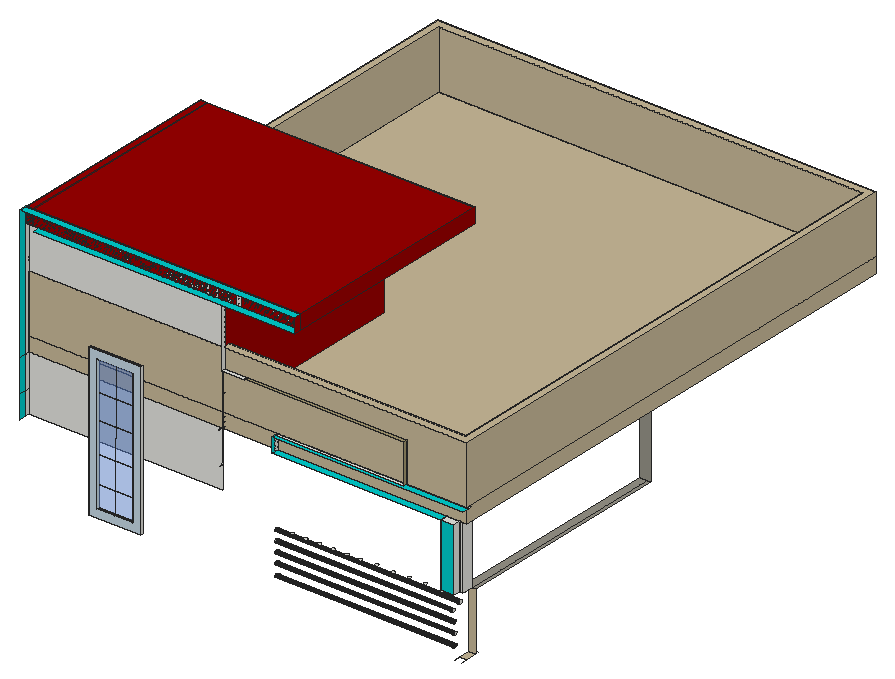
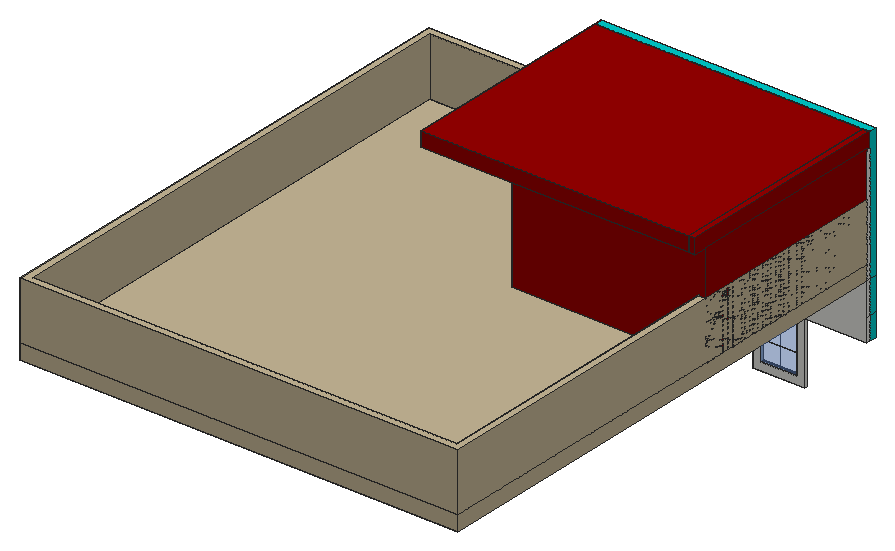
# SketchUp Ruby script. Lengths in inches.
U = 1.inch
M = Sketchup.active_model
def pt(a) = Geom::Point3d.new(a.map { |v| v * U })
def face(e, loops, mat)
  f = e.add_face(loops[0].map { |a| pt(a) })
  loops[1..].each { |l| e.add_face(l.map { |a| pt(a) }).erase! }
  f.material = f.back_material = mat if mat
  f
end
# faces: each face lists its corners as indices into pts; further lists are holes
def faces(e, pts, list, mat = nil) = list.each { |f| face(e, (f[0].is_a?(Array) ? f : [f]).map { |l| l.map { |i| pts[i] } }, mat) }
# xy, xz, yz: faces in a plane at the given z, y or x. An outline is a flat list of corners, or four numbers for a rectangle; further outlines are holes
def ring(l) = l.size == 4 ? [[l[0], l[1]], [l[2], l[1]], [l[2], l[3]], [l[0], l[3]]] : l.each_slice(2).to_a
def flat(e, list, mat, &to3) = list.each { |f| face(e, (f[0].is_a?(Array) ? f : [f]).map { |l| ring(l).map { |u, v| to3.(u, v) } }, mat) }
def xy(e, z, list, mat = nil) = flat(e, list, mat) { |x, y| [x, y, z] }
def xz(e, y, list, mat = nil) = flat(e, list, mat) { |x, z| [x, y, z] }
def yz(e, x, list, mat = nil) = flat(e, list, mat) { |y, z| [x, y, z] }
def lines(e, pts, list) = list.each { |a, b| e.add_line(pt(pts[a]), pt(pts[b])) }
# prism: a flat outline (further loops are holes) pulled along v
def prism(e, loops, v, mat = nil)
  f = face(e, loops, mat); d = Geom::Vector3d.new(v.map { |x| x * U })
  f.pushpull(f.normal.samedirection?(d) ? d.length : -d.length)
end
def box(e, o, s, mat = nil) = prism(e, [[o, [o[0] + s[0], o[1], o[2]], [o[0] + s[0], o[1] + s[1], o[2]], [o[0], o[1] + s[1], o[2]]]], [0, 0, s[2]], mat)
def at(x, y, z, deg = 0) = Geom::Transformation.translation(pt([x, y, z])) * Geom::Transformation.rotation(ORIGIN, Z_AXIS, deg.degrees)
def axes(o, x, y, z) = Geom::Transformation.new([*x, 0, *y, 0, *z, 0, *pt(o).to_a, 1])
def part(name) = M.definitions.add(name)
# library, detail: a bought-in or finely detailed component or shape, given as its bounding box
def library(name, o, s) = part(name).tap { |d| box(d.entities, o, s) }
def detail(e, o, s) = box(e.add_group.entities, o, s)
def put(e, d, t, mat = nil) = e.add_instance(d, t).tap { |i| i.material = mat if mat }
def group(e, t, mat = nil) = e.add_group.tap { |g| g.transformation = t; g.material = mat if mat }.entities
root = M.entities
M.materials.add("[Color A07]").color = [153, 0, 0]
M.materials.add("[Color B03]").color = [255, 140, 101]
M.materials.add("[Color H06]").color = [0, 204, 204]
M.materials.add("[Formica Beige]").color = [211, 187, 149]
M.materials.add("[Formica Graystone]").color = [149, 146, 135]
M.materials.add("[Quartz Light Brown]").color = [199, 184, 152]
M.materials.add("[Terrazzo Light Blue]").color = [196, 214, 227]
M.materials.add("[Translucent Glass Blue]").color = [100, 149, 237]
M.materials["[Translucent Glass Blue]"].alpha = 0.5
M.materials.add("[Translucent Glass Gray]1").color = [128, 128, 128]
M.materials["[Translucent Glass Gray]1"].alpha = 0.5
M.materials.add("[Wood Lumber ButtJoined]").color = [164, 152, 112]
c1 = part("Group\#7")
xy(c1.entities,0,[[0,0,32.48,1.97]])
xy(c1.entities,0.98,[[0.98,0,31.5,0.98],[0.98,0.98,31.5,1.97]])
xy(c1.entities,8.86,[[0.98,0,31.5,0.98],[0.98,0.98,31.5,1.97]])
xy(c1.entities,9.84,[[0,0,32.48,1.97]])
xz(c1.entities,0,[[[0,0,32.48,9.84],[0.98,0.98,31.5,8.86]]])
xz(c1.entities,0.98,[[0.98,0.98,31.5,8.86]],"[Translucent Glass Gray]1")
xz(c1.entities,1.97,[[[0,0,32.48,9.84],[0.98,0.98,31.5,8.86]]])
yz(c1.entities,0,[[0,0,1.97,9.84]])
yz(c1.entities,0.98,[[0,0.98,0.98,8.86],[0.98,0.98,1.97,8.86]])
yz(c1.entities,31.5,[[0,0.98,0.98,8.86],[0.98,0.98,1.97,8.86]])
yz(c1.entities,32.48,[[0,0,1.97,9.84]])
c2 = part("Group\#9")
xy(c2.entities,0,[[0,0,32.48,1.97]])
xy(c2.entities,0.98,[[0.98,0,31.5,0.98],[0.98,0.98,31.5,1.97]])
xy(c2.entities,71.85,[[0.98,0,31.5,0.98],[0.98,0.98,31.5,1.97]])
xy(c2.entities,72.83,[[0,0,32.48,1.97]])
xz(c2.entities,0,[[[0,0,32.48,72.83],[0.98,0.98,31.5,71.85]]])
xz(c2.entities,0.98,[[0.98,0.98,31.5,71.85]],"[Translucent Glass Gray]1")
xz(c2.entities,1.97,[[[0,0,32.48,72.83],[0.98,0.98,31.5,71.85]]])
yz(c2.entities,0,[[0,0,1.97,72.83]])
yz(c2.entities,0.98,[[0,0.98,0.98,71.85],[0.98,0.98,1.97,71.85]])
yz(c2.entities,31.5,[[0,0.98,0.98,71.85],[0.98,0.98,1.97,71.85]])
yz(c2.entities,32.48,[[0,0,1.97,72.83]])
c3 = part("FIXED+GLASS+WINDOW+WITH+TRANSOM")
g1 = group(c3.entities,at(0,0,0))
xy(g1,0,[[0,0,70.86,3.9375]])
xy(g1,1.97,[[1.97,0,34.45,0.98],[36.42,0,68.9,3.9375],[1.97,2.95,34.45,3.9375]])
xy(g1,86.61,[[1.97,0,34.45,3.9375],[34.45,0,36.42,3.9375],[36.42,0,68.9,3.9375]])
xy(g1,88.58,[[0,0,70.86,3.9375]])
xz(g1,0,[[[0,0,70.86,88.58],[1.97,1.97,34.45,86.61],[36.42,1.97,68.9,86.61]]])
xz(g1,3.9375,[[[0,0,70.86,88.58],[1.97,1.97,34.45,86.61],[36.42,1.97,68.9,86.61]]])
yz(g1,0,[[0,0,3.9375,88.58]])
yz(g1,1.97,[[0,1.97,3.9375,74.8],[0,76.77,3.9375,86.61]])
yz(g1,34.45,[[0,1.97,3.9375,86.61]])
yz(g1,36.42,[[0,1.97,3.9375,86.61]])
yz(g1,68.9,[[0,1.97,3.9375,86.61]])
yz(g1,70.86,[[0,0,3.9375,88.58]])
g2 = group(g1,at(1.97,0,74.8))
box(g2,[0,0,0],[66.93,3.9375,1.97])
put(g1,c1,at(1.97,0.98,76.77))
put(g1,c1,at(36.42,0.98,76.77))
put(g1,c2,at(1.97,0.98,1.97))
put(g1,c2,at(36.42,0.98,1.97))
xy(root,140.125,[[438.6,84.38,444.38,93.38]],"[Quartz Light Brown]")
xy(root,141.25,[[137.82,79.38,180.63,81.38]])
xy(root,147.98,[[144.54,79.38,173.9,81.38]],"[Terrazzo Light Blue]")
xy(root,164.61,[[274.3,273.125,322.3,279.65]],"[Formica Graystone]")
xy(root,184.375,[[302.87,81.02,303.14,81.06,303.4,81.16,303.62,81.33,303.79,81.55,303.89,81.81,303.93,82.08,303.89,82.36,303.79,82.61,303.62,82.83,303.4,83,303.14,83.11,302.87,83.15,302.59,83.11,302.34,83,302.12,82.83,301.95,82.61,301.84,82.36,301.81,82.08,301.84,81.81,301.95,81.55,302.12,81.33,302.34,81.16,302.59,81.06],[314.06,81.02,314.33,81.06,314.59,81.16,314.81,81.33,314.98,81.55,315.08,81.81,315.12,82.08,315.08,82.36,314.98,82.61,314.81,82.83,314.59,83,314.33,83.11,314.06,83.15,313.78,83.11,313.52,83,313.3,82.83,313.13,82.61,313.03,82.36,312.99,82.08,313.03,81.81,313.13,81.55,313.3,81.33,313.52,81.16,313.78,81.06]])
xy(root,184.625,[[325.24,81.02,325.52,81.06,325.77,81.16,325.99,81.33,326.16,81.55,326.27,81.81,326.31,82.08,326.27,82.36,326.16,82.61,325.99,82.83,325.77,83,325.52,83.11,325.24,83.15,324.97,83.11,324.71,83,324.49,82.83,324.32,82.61,324.22,82.36,324.18,82.08,324.22,81.81,324.32,81.55,324.49,81.33,324.71,81.16,324.97,81.06],[336.43,81.02,336.71,81.06,336.96,81.16,337.18,81.33,337.35,81.55,337.46,81.81,337.49,82.08,337.46,82.36,337.35,82.61,337.18,82.83,336.96,83,336.71,83.11,336.43,83.15,336.16,83.11,335.9,83,335.68,82.83,335.51,82.61,335.4,82.36,335.37,82.08,335.4,81.81,335.51,81.55,335.68,81.33,335.9,81.16,336.16,81.06],[347.62,81.02,347.89,81.06,348.15,81.16,348.37,81.33,348.54,81.55,348.64,81.81,348.68,82.08,348.64,82.36,348.54,82.61,348.37,82.83,348.15,83,347.89,83.11,347.62,83.15,347.34,83.11,347.09,83,346.87,82.83,346.7,82.61,346.59,82.36,346.56,82.08,346.59,81.81,346.7,81.55,346.87,81.33,347.09,81.16,347.34,81.06]])
xy(root,184.75,[[358.81,81.02,359.08,81.06,359.34,81.16,359.56,81.33,359.73,81.55,359.83,81.81,359.87,82.08,359.83,82.36,359.73,82.61,359.56,82.83,359.34,83,359.08,83.11,358.81,83.15,358.53,83.11,358.27,83,358.05,82.83,357.88,82.61,357.78,82.36,357.74,82.08,357.78,81.81,357.88,81.55,358.05,81.33,358.27,81.16,358.53,81.06]])
xy(root,184.9375,[[385.56,81.02,385.83,81.06,386.09,81.16,386.31,81.33,386.48,81.55,386.58,81.81,386.62,82.08,386.58,82.36,386.48,82.61,386.31,82.83,386.09,83,385.83,83.11,385.56,83.15,385.28,83.11,385.02,83,384.8,82.83,384.63,82.61,384.53,82.36,384.49,82.08,384.53,81.81,384.63,81.55,384.8,81.33,385.02,81.16,385.28,81.06]])
xy(root,185.3125,[[425.68,81.02,425.96,81.06,426.21,81.16,426.43,81.33,426.6,81.55,426.71,81.81,426.74,82.08,426.71,82.36,426.6,82.61,426.43,82.83,426.21,83,425.96,83.11,425.68,83.15,425.41,83.11,425.15,83,424.93,82.83,424.76,82.61,424.65,82.36,424.62,82.08,424.65,81.81,424.76,81.55,424.93,81.33,425.15,81.16,425.41,81.06]])
xy(root,185.5625,[[372.18,81.02,372.46,81.06,372.71,81.16,372.93,81.33,373.1,81.55,373.21,81.81,373.24,82.08,373.21,82.36,373.1,82.61,372.93,82.83,372.71,83,372.46,83.11,372.18,83.15,371.91,83.11,371.65,83,371.43,82.83,371.26,82.61,371.15,82.36,371.12,82.08,371.15,81.81,371.26,81.55,371.43,81.33,371.65,81.16,371.91,81.06]])
xy(root,185.625,[[398.93,81.02,399.21,81.06,399.46,81.16,399.68,81.33,399.85,81.55,399.96,81.81,399.99,82.08,399.96,82.36,399.85,82.61,399.68,82.83,399.46,83,399.21,83.11,398.93,83.15,398.66,83.11,398.4,83,398.18,82.83,398.01,82.61,397.9,82.36,397.87,82.08,397.9,81.81,398.01,81.55,398.18,81.33,398.4,81.16,398.66,81.06]])
xy(root,185.8125,[[412.31,81.02,412.58,81.06,412.84,81.16,413.06,81.33,413.23,81.55,413.33,81.81,413.37,82.08,413.33,82.36,413.23,82.61,413.06,82.83,412.84,83,412.58,83.11,412.31,83.15,412.03,83.11,411.77,83,411.55,82.83,411.38,82.61,411.28,82.36,411.24,82.08,411.28,81.81,411.38,81.55,411.55,81.33,411.77,81.16,412.03,81.06]])
xy(root,188,[[427.85,78.76,435.38,84.38],[435.38,78.76,438.6,84.38],[435.38,84.38,438.6,86.51],[438.6,84.38,441.16,86.51],[438.6,86.51,441.16,93.38],
  [441.16,86.51,441.2,93.38]])
xy(root,188,[[435.38,86.51,438.6,86.51,438.6,93.38,441.2,93.38,441.2,273.125,435.38,273.125],[441.2,93.38,444.38,273.125]],"[Formica Graystone]")
xy(root,204,[[357.88,273.125,393.88,279.65]])
xy(root,212.61,[[274.3,273.125,322.3,279.65]],"[Formica Graystone]")
xy(root,240,[[427.85,78.76,438.6,84.38],[243.32,81.38,243.82,84.38],[243.82,84.38,264.38,84.38,264.38,93.38,93.38,93.38,93.38,495.38,435.38,495.38,435.38,273.125,444.38,273.125,444.38,504.38,84.38,504.38,84.38,84.57,243.82,84.57],[84.38,84.38,243.32,84.57],[243.32,84.38,243.82,84.57],
  [427.85,84.38,438.6,86.51],[438.6,84.38,441.16,93.38]])
xy(root,240,[[93.38,273.125,435.38,279.65]],"[Color B03]")
xy(root,240,[[288.89,78.76,427.85,84.38],[288.89,84.38,427.85,86.51],[288.89,86.51,438.6,93.38]],"[Color H06]")
xy(root,252,[[288.89,81.38,394.7,84.38],[[84.38,84.38,243.82,250.01],[90.38,90.38,237.32,244.01]],[288.89,84.38,445.9,86.51],[90.38,90.38,237.32,244.01]])
xy(root,252,[[288.89,78.76,445.9,78.76,445.9,84.38,394.7,84.38,394.7,81.38,288.89,81.38]],"[Color H06]")
xy(root,258.08,[[144.54,79.38,173.9,81.38]],"[Terrazzo Light Blue]")
xy(root,264.8125,[[137.82,79.38,180.63,81.38]])
xy(root,284.5,[[245.63,81.38,264.38,84.38],[243.82,84.38,245.63,84.57]])
xy(root,284.625,[[264.38,81.38,394.7,84.38]],"[Wood Lumber ButtJoined]")
xy(root,336.625,[[84.38,81.38,245.63,84.38],[84.38,84.38,245.63,84.57]])
xy(root,336.625,[[95.53,75.38,310.04,81.38]],"[Color H06]")
xy(root,337,[[[84.38,84.38,243.82,250.01],[90.38,90.38,237.32,244.01]]])
xy(root,348.625,[[84.38,75.38,310.04,81.38]],"[Color H06]")
xz(root,78.76,[[427.85,188,438.6,240]],"[Color H06]")
xz(root,79.38,[[[137.82,141.25,180.63,264.8125],[144.54,147.98,173.9,258.08]]],"[Terrazzo Light Blue]")
xz(root,81.38,[[[137.82,141.25,180.63,264.8125],[144.54,147.98,173.9,258.08]],[84.38,336.625,310.04,348.625]])
xz(root,81.38,[[144.54,147.98,173.9,164.85],[144.54,164.85,173.9,186.92],[144.54,186.92,173.9,211.79],[144.54,211.79,173.9,232.45],[144.54,232.45,173.9,258.08]],"[Translucent Glass Blue]")
xz(root,84.38,[[427.85,188,438.6,240],[438.6,188,441.16,240],[84.38,194.4375,84.38,240,243.32,240,243.32,213.125,243.82,213.125,243.82,194.4375],[243.32,213.125,243.82,240],[84.38,240,243.82,252],
  [243.82,240,243.82,284.5,245.63,284.5,245.26,240],[245.26,240,245.63,284.5,245.63,240],[84.38,252,243.82,336.625],[243.82,284.5,245.63,336.625],[84.38,336.625,243.82,337]])
xz(root,84.57,[[84.38,240,84.38,336.625,245.63,336.625,245.63,284.5,243.82,284.5,243.82,240]])
xz(root,90.38,[[90.38,252,237.32,337]])
xz(root,93.38,[[438.6,188,441.16,240]])
xz(root,93.38,[[438.6,140.125,444.38,188]],"[Quartz Light Brown]")
xz(root,244.01,[[90.38,252,237.32,337]])
xz(root,250.01,[[84.38,252,243.82,337]],"[Color A07]")
xz(root,273.125,[[435.38,188,444.38,240]],"[Formica Graystone]")
yz(root,84.38,[[81.38,194.4375,84.38,213.125],[81.38,213.125,84.38,240],[81.38,240,84.38,336.625],[84.38,240,84.57,252],[84.38,252,84.57,336.625],
  [84.38,336.625,84.57,337]])
yz(root,84.38,[[84.57,252,250.01,337]],"[Color A07]")
yz(root,84.38,[[75.38,194.4375,81.38,213.125],[75.38,213.125,81.38,240],[75.38,240,81.38,348.625]],"[Color H06]")
yz(root,90.38,[[90.38,252,244.01,337]])
yz(root,137.82,[[79.38,141.25,81.38,264.8125]])
yz(root,144.54,[[79.38,147.98,81.38,258.08]],"[Terrazzo Light Blue]")
yz(root,173.9,[[79.38,147.98,81.38,258.08]],"[Terrazzo Light Blue]")
yz(root,180.63,[[79.38,141.25,81.38,264.8125]])
yz(root,237.32,[[90.38,252,244.01,337]])
yz(root,243.82,[[84.38,240,84.57,252],[84.38,252,84.57,284.5]])
yz(root,243.82,[[84.57,252,250.01,252,250.01,337,84.38,337,84.38,284.5,84.57,284.5]],"[Color A07]")
yz(root,245.63,[[81.38,284.5,84.38,336.625],[84.38,284.5,84.57,336.625]])
yz(root,264.38,[[81.38,284.5,84.38,284.625]])
yz(root,274.3,[[273.125,164.61,279.65,212.61]],"[Formica Graystone]")
yz(root,288.89,[[83.14,156.08,82.83,156.12,82.54,156.23,82.3,156.42,82.11,156.67,81.99,156.96,81.95,157.26,81.99,157.57,82.11,157.86,82.3,158.1,82.54,158.29,82.83,158.41,83.14,158.45,83.44,158.41,83.73,158.29,83.98,158.1,84.17,157.86,84.28,157.57,84.33,157.26,84.28,156.96,84.17,156.67,83.98,156.42,83.73,156.23,83.44,156.12],[83.14,164.26,82.83,164.3,82.54,164.42,82.3,164.61,82.11,164.86,81.99,165.14,81.95,165.45,81.99,165.76,82.11,166.04,82.3,166.29,82.54,166.48,82.83,166.6,83.14,166.64,83.44,166.6,83.73,166.48,83.98,166.29,84.17,166.04,84.28,165.76,84.33,165.45,84.28,165.14,84.17,164.86,83.98,164.61,83.73,164.42,83.44,164.3],[83.14,172.45,82.83,172.49,82.54,172.61,82.3,172.8,82.11,173.04,81.99,173.33,81.95,173.64,81.99,173.95,82.11,174.23,82.3,174.48,82.54,174.67,82.83,174.78,83.14,174.83,83.44,174.78,83.73,174.67,83.98,174.48,84.17,174.23,84.28,173.95,84.33,173.64,84.28,173.33,84.17,173.04,83.98,172.8,83.73,172.61,83.44,172.49],[83.14,180.64,82.83,180.68,82.54,180.8,82.3,180.99,82.11,181.23,81.99,181.52,81.95,181.83,81.99,182.13,82.11,182.42,82.3,182.67,82.54,182.85,82.83,182.97,83.14,183.01,83.44,182.97,83.73,182.85,83.98,182.67,84.17,182.42,84.28,182.13,84.33,181.83,84.28,181.52,84.17,181.23,83.98,180.99,83.73,180.8,83.44,180.68],[81.38,240,84.38,252],
  [84.38,240,86.51,252],[86.51,240,93.38,252]])
yz(root,288.89,[[78.76,240,81.38,252]],"[Color H06]")
yz(root,310.04,[[75.38,336.625,81.38,348.625]],"[Color A07]")
yz(root,322.3,[[273.125,164.61,279.65,212.61]],"[Formica Graystone]")
yz(root,394.7,[[84.38,252,85.76,283.5625]])
yz(root,394.7,[[81.38,252,84.38,284.625]],"[Wood Lumber ButtJoined]")
yz(root,427.85,[[78.76,188,84.38,240]],"[Color H06]")
yz(root,434.77,[[83.14,172.45,83.44,172.49,83.73,172.61,83.98,172.8,84.17,173.04,84.28,173.33,84.33,173.64,84.28,173.95,84.17,174.23,83.98,174.48,83.73,174.67,83.44,174.78,83.14,174.83,82.83,174.78,82.54,174.67,82.3,174.48,82.11,174.23,81.99,173.95,81.95,173.64,81.99,173.33,82.11,173.04,82.3,172.8,82.54,172.61,82.83,172.49]])
yz(root,436.08,[[83.14,156.08,83.44,156.12,83.73,156.23,83.98,156.42,84.17,156.67,84.28,156.96,84.33,157.26,84.28,157.57,84.17,157.86,83.98,158.1,83.73,158.29,83.44,158.41,83.14,158.45,82.83,158.41,82.54,158.29,82.3,158.1,82.11,157.86,81.99,157.57,81.95,157.26,81.99,156.96,82.11,156.67,82.3,156.42,82.54,156.23,82.83,156.12]])
yz(root,438.6,[[78.76,188,84.38,240],[84.38,188,86.51,240]])
yz(root,438.6,[[86.51,188,93.38,240]],"[Color H06]")
yz(root,440.33,[[83.14,180.64,83.44,180.68,83.73,180.8,83.98,180.99,84.17,181.23,84.28,181.52,84.33,181.83,84.28,182.13,84.17,182.42,83.98,182.67,83.73,182.85,83.44,182.97,83.14,183.01,82.83,182.97,82.54,182.85,82.3,182.67,82.11,182.42,81.99,182.13,81.95,181.83,81.99,181.52,82.11,181.23,82.3,180.99,82.54,180.8,82.83,180.68]])
yz(root,441.16,[[84.38,188,93.38,240]])
p = [[288.89,82.54,147.05],[288.89,82.83,146.93],[436.08,82.83,146.93],[436.08,82.54,147.05],[288.89,83.14,146.89],[436.08,83.14,146.89],
  [288.89,83.44,146.93],[436.08,83.44,146.93],[288.89,83.73,147.05],[436.08,83.73,147.05],[288.89,82.3,147.24],[436.08,82.3,147.24],
  [288.89,83.98,147.24],[436.08,83.98,147.24],[288.89,82.11,147.48],[436.08,82.11,147.48],[288.89,84.17,147.48],[436.08,84.17,147.48],
  [288.89,81.99,147.77],[436.08,81.99,147.77],[288.89,84.28,147.77],[436.08,84.28,147.77],[288.89,81.95,148.08],[436.08,81.95,148.08],
  [288.89,84.33,148.08],[436.08,84.33,148.08],[288.89,81.99,148.38],[436.08,81.99,148.38],[288.89,84.28,148.38],[436.08,84.28,148.38],
  [288.89,82.11,148.67],[436.08,82.11,148.67],[288.89,84.17,148.67],[436.08,84.17,148.67],[288.89,82.3,148.92],[436.08,82.3,148.92],
  [288.89,83.98,148.92],[436.08,83.98,148.92],[288.89,82.54,149.1],[436.08,82.54,149.1],[288.89,83.73,149.1],[436.08,83.73,149.1],
  [288.89,82.83,149.22],[436.08,82.83,149.22],[288.89,83.44,149.22],[436.08,83.44,149.22],[288.89,83.14,149.26],[436.08,83.14,149.26],
  [288.89,82.54,156.23],[288.89,82.83,156.12],[436.08,82.83,156.12],[436.08,82.54,156.23],[288.89,83.14,156.08],[436.08,83.14,156.08],
  [288.89,83.44,156.12],[436.08,83.44,156.12],[288.89,83.73,156.23],[436.08,83.73,156.23],[288.89,82.3,156.42],[436.08,82.3,156.42],
  [288.89,83.98,156.42],[436.08,83.98,156.42],[288.89,82.11,156.67],[436.08,82.11,156.67],[288.89,84.17,156.67],[436.08,84.17,156.67],
  [288.89,81.99,156.96],[436.08,81.99,156.96],[288.89,84.28,156.96],[436.08,84.28,156.96],[288.89,81.95,157.26],[436.08,81.95,157.26],
  [288.89,84.33,157.26],[436.08,84.33,157.26],[288.89,81.99,157.57],[436.08,81.99,157.57],[288.89,84.28,157.57],[436.08,84.28,157.57],
  [288.89,82.11,157.86],[436.08,82.11,157.86],[288.89,84.17,157.86],[436.08,84.17,157.86],[288.89,82.3,158.1],[436.08,82.3,158.1],
  [288.89,83.98,158.1],[436.08,83.98,158.1],[288.89,82.54,158.29],[436.08,82.54,158.29],[288.89,83.73,158.29],[436.08,83.73,158.29],
  [288.89,82.83,158.41],[436.08,82.83,158.41],[288.89,83.44,158.41],[436.08,83.44,158.41],[288.89,83.14,158.45],[436.08,83.14,158.45],
  [288.89,82.54,164.42],[288.89,82.83,164.3],[435.38,82.83,164.3],[435.38,82.54,164.42],[288.89,83.14,164.26],[435.38,83.14,164.26],
  [288.89,83.44,164.3],[435.38,83.44,164.3],[288.89,83.73,164.42],[435.38,83.73,164.42],[288.89,82.3,164.61],[435.38,82.3,164.61],
  [288.89,83.98,164.61],[435.38,83.98,164.61],[288.89,82.11,164.86],[435.38,82.11,164.86],[288.89,84.17,164.86],[435.38,84.17,164.86],
  [288.89,81.99,165.14],[435.38,81.99,165.14],[288.89,84.28,165.14],[435.38,84.28,165.14],[288.89,81.95,165.45],[435.38,81.95,165.45],
  [288.89,84.33,165.45],[435.38,84.33,165.45],[288.89,81.99,165.76],[435.38,81.99,165.76],[288.89,84.28,165.76],[435.38,84.28,165.76],
  [288.89,82.11,166.04],[435.38,82.11,166.04],[288.89,84.17,166.04],[435.38,84.17,166.04],[288.89,82.3,166.29],[435.38,82.3,166.29],
  [288.89,83.98,166.29],[435.38,83.98,166.29],[288.89,82.54,166.48],[435.38,82.54,166.48],[288.89,83.73,166.48],[435.38,83.73,166.48],
  [288.89,82.83,166.6],[435.38,82.83,166.6],[288.89,83.44,166.6],[435.38,83.44,166.6],[288.89,83.14,166.64],[435.38,83.14,166.64],
  [288.89,82.54,172.61],[288.89,82.83,172.49],[434.77,82.83,172.49],[434.77,82.54,172.61],[288.89,83.14,172.45],[434.77,83.14,172.45],
  [288.89,83.44,172.49],[434.77,83.44,172.49],[288.89,83.73,172.61],[434.77,83.73,172.61],[288.89,82.3,172.8],[434.77,82.3,172.8],
  [288.89,83.98,172.8],[434.77,83.98,172.8],[288.89,82.11,173.04],[434.77,82.11,173.04],[288.89,84.17,173.04],[434.77,84.17,173.04],
  [288.89,81.99,173.33],[434.77,81.99,173.33],[288.89,84.28,173.33],[434.77,84.28,173.33],[288.89,81.95,173.64],[434.77,81.95,173.64],
  [288.89,84.33,173.64],[434.77,84.33,173.64],[288.89,81.99,173.95],[434.77,81.99,173.95],[288.89,84.28,173.95],[434.77,84.28,173.95],
  [288.89,82.11,174.23],[434.77,82.11,174.23],[288.89,84.17,174.23],[434.77,84.17,174.23],[288.89,82.3,174.48],[434.77,82.3,174.48],
  [288.89,83.98,174.48],[434.77,83.98,174.48],[288.89,82.54,174.67],[434.77,82.54,174.67],[288.89,83.73,174.67],[434.77,83.73,174.67],
  [288.89,82.83,174.78],[434.77,82.83,174.78],[288.89,83.44,174.78],[434.77,83.44,174.78],[288.89,83.14,174.83],[434.77,83.14,174.83],
  [288.89,82.83,180.68],[288.89,83.14,180.64],[440.33,83.14,180.64],[440.33,82.83,180.68],[288.89,83.44,180.68],[440.33,83.44,180.68],
  [288.89,82.54,180.8],[440.33,82.54,180.8],[288.89,83.73,180.8],[440.33,83.73,180.8],[288.89,82.3,180.99],[440.33,82.3,180.99],
  [288.89,83.98,180.99],[440.33,83.98,180.99],[288.89,82.11,181.23],[440.33,82.11,181.23],[288.89,84.17,181.23],[440.33,84.17,181.23],
  [288.89,81.99,181.52],[440.33,81.99,181.52],[288.89,84.28,181.52],[440.33,84.28,181.52],[288.89,81.95,181.83],[440.33,81.95,181.83],
  [288.89,84.33,181.83],[440.33,84.33,181.83],[288.89,81.99,182.13],[440.33,81.99,182.13],[288.89,84.28,182.13],[440.33,84.28,182.13],
  [288.89,82.11,182.42],[440.33,82.11,182.42],[288.89,84.17,182.42],[440.33,84.17,182.42],[288.89,82.3,182.67],[440.33,82.3,182.67],
  [288.89,83.98,182.67],[440.33,83.98,182.67],[288.89,82.54,182.85],[440.33,82.54,182.85],[288.89,83.73,182.85],[440.33,83.73,182.85],
  [288.89,82.83,182.97],[440.33,82.83,182.97],[288.89,83.44,182.97],[440.33,83.44,182.97],[288.89,83.14,183.01],[440.33,83.14,183.01],
  [444.38,96.7,140.125],[438.6,96.7,140.125],[438.6,96.7,188],[444.38,78.76,140.125],[444.38,84.38,140.125],[438.6,78.76,140.125],
  [438.6,84.38,140.125],[438.6,93.38,140.125],[245.63,84.38,240],[245.63,81.38,240],[243.32,84.38,213.125],[243.32,81.38,213.125],
  [243.82,84.38,213.125],[243.82,81.38,213.125],[159.22,81.38,258.08],[159.22,79.38,147.98]]
faces(root,p,[[0,1,2,3],[1,4,5,2],[4,6,7,5],[6,8,9,7],[10,0,3,11],[8,12,13,9],[14,10,11,15],[12,16,17,13],
  [18,14,15,19],[16,20,21,17],[22,18,19,23],[20,24,25,21],[26,22,23,27],[24,28,29,25],[30,26,27,31],[28,32,33,29],
  [34,30,31,35],[32,36,37,33],[38,34,35,39],[36,40,41,37],[42,38,39,43],[40,44,45,41],[46,42,43,47],[44,46,47,45],
  [48,49,50,51],[49,52,53,50],[52,54,55,53],[54,56,57,55],[58,48,51,59],[56,60,61,57],[62,58,59,63],[60,64,65,61],
  [66,62,63,67],[64,68,69,65],[70,66,67,71],[68,72,73,69],[74,70,71,75],[72,76,77,73],[78,74,75,79],[76,80,81,77],
  [82,78,79,83],[80,84,85,81],[86,82,83,87],[84,88,89,85],[90,86,87,91],[88,92,93,89],[94,90,91,95],[92,94,95,93],
  [96,97,98,99],[97,100,101,98],[100,102,103,101],[102,104,105,103],[106,96,99,107],[104,108,109,105],[110,106,107,111],[108,112,113,109],
  [114,110,111,115],[112,116,117,113],[118,114,115,119],[116,120,121,117],[122,118,119,123],[120,124,125,121],[126,122,123,127],[124,128,129,125],
  [130,126,127,131],[128,132,133,129],[134,130,131,135],[132,136,137,133],[138,134,135,139],[136,140,141,137],[142,138,139,143],[140,142,143,141],
  [144,145,146,147],[145,148,149,146],[148,150,151,149],[150,152,153,151],[154,144,147,155],[152,156,157,153],[158,154,155,159],[156,160,161,157],
  [162,158,159,163],[160,164,165,161],[166,162,163,167],[164,168,169,165],[170,166,167,171],[168,172,173,169],[174,170,171,175],[172,176,177,173],
  [178,174,175,179],[176,180,181,177],[182,178,179,183],[180,184,185,181],[186,182,183,187],[184,188,189,185],[190,186,187,191],[188,190,191,189],
  [192,193,194,195],[193,196,197,194],[198,192,195,199],[196,200,201,197],[202,198,199,203],[200,204,205,201],[206,202,203,207],[204,208,209,205],
  [210,206,207,211],[208,212,213,209],[214,210,211,215],[212,216,217,213],[218,214,215,219],[216,220,221,217],[222,218,219,223],[220,224,225,221],
  [226,222,223,227],[224,228,229,225],[230,226,227,231],[228,232,233,229],[234,230,231,235],[232,236,237,233],[238,234,235,239],[236,238,239,237]],"[Formica Beige]")
lines(root,p,[[240,241],[242,241],[243,244],[245,246],[247,241],[248,249],[250,251],[252,253],[254,255]])
put(root,c3,axes([274.3,272.95,164.61],[0.67815,0,0],[0,0.53715,0],[0,0,0.53715]))
g3 = group(root,at(84.38,84.38,240),"[Quartz Light Brown]")
xy(g3,0,[[0,0,360,420]])
xy(g3,12,[[[0,0,360,420],[6,6,354,414]],[6,6,354,414]])
xy(g3,60,[[[0,0,360,420],[6,6,354,414]]])
xz(g3,0,[[0,0,360,12],[0,12,360,60]])
xz(g3,6,[[6,12,354,60]])
xz(g3,414,[[6,12,354,60]])
xz(g3,420,[[0,0,360,12],[0,12,360,60]])
yz(g3,0,[[0,0,420,12],[0,12,420,60]])
yz(g3,6,[[6,12,414,60]])
yz(g3,354,[[6,12,414,60]])
yz(g3,360,[[0,0,420,12],[0,12,420,60]])
g4 = group(root,at(91.04,81.38,336.625),"[Color A07]")
xy(g4,0,[[-6.28,0,-0.66,178.9375],[-0.66,0,219.0625,178.9375]])
xy(g4,12,[[-6.28,0,-0.66,178.9375],[-0.66,0,219.0625,178.9375]])
xz(g4,0,[[-6.28,0,-0.66,12],[-0.66,0,219.0625,12]])
xz(g4,178.9375,[[-6.28,0,-0.66,12],[-0.66,0,219.0625,12]])
yz(g4,-6.28,[[0,0,178.9375,12]])
yz(g4,-0.66,[[0,0,178.9375,12]])
yz(g4,219.0625,[[0,0,178.9375,12]])
